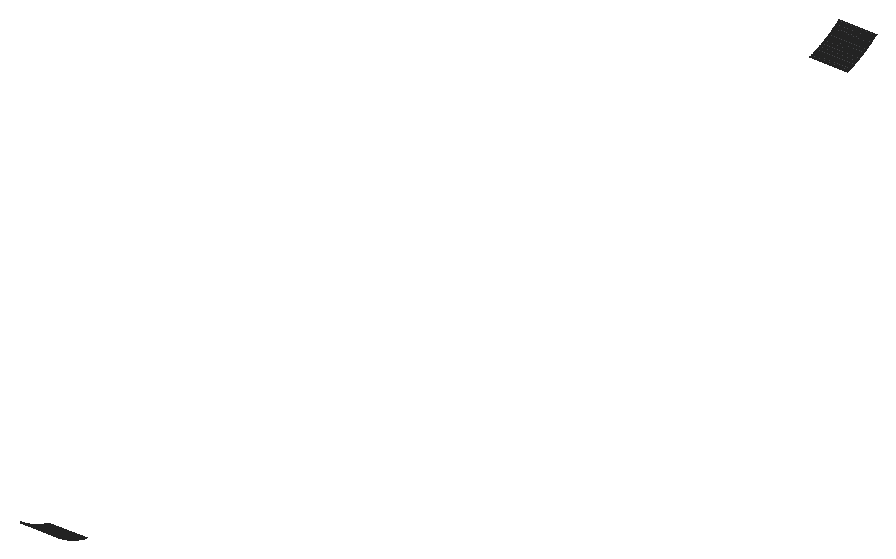
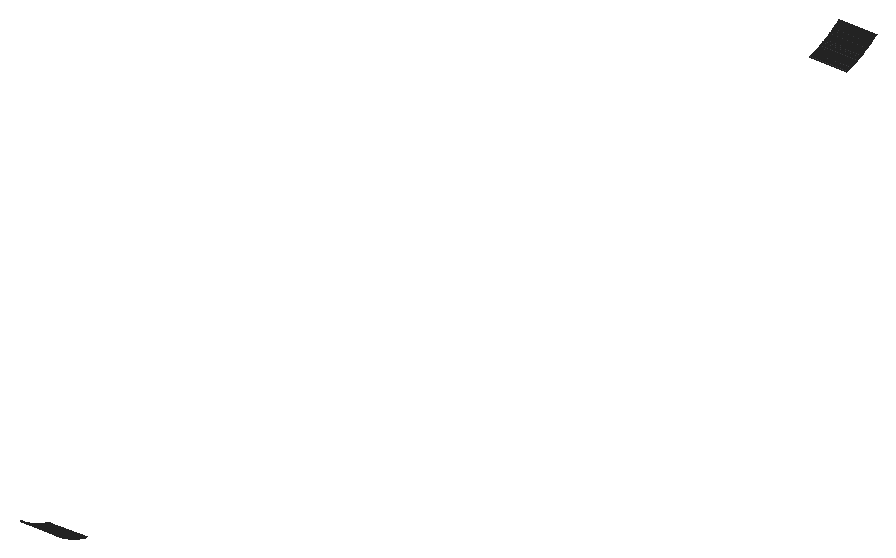
# SketchUp Ruby script. Lengths in inches.
U = 1.inch
M = Sketchup.active_model
def pt(a) = Geom::Point3d.new(a.map { |v| v * U })
def face(e, loops, mat)
  f = e.add_face(loops[0].map { |a| pt(a) })
  loops[1..].each { |l| e.add_face(l.map { |a| pt(a) }).erase! }
  f.material = f.back_material = mat if mat
  f
end
# faces: each face lists its corners as indices into pts; further lists are holes
def faces(e, pts, list, mat = nil) = list.each { |f| face(e, (f[0].is_a?(Array) ? f : [f]).map { |l| l.map { |i| pts[i] } }, mat) }
# xy, xz, yz: faces in a plane at the given z, y or x. An outline is a flat list of corners, or four numbers for a rectangle; further outlines are holes
def ring(l) = l.size == 4 ? [[l[0], l[1]], [l[2], l[1]], [l[2], l[3]], [l[0], l[3]]] : l.each_slice(2).to_a
def flat(e, list, mat, &to3) = list.each { |f| face(e, (f[0].is_a?(Array) ? f : [f]).map { |l| ring(l).map { |u, v| to3.(u, v) } }, mat) }
def xy(e, z, list, mat = nil) = flat(e, list, mat) { |x, y| [x, y, z] }
def xz(e, y, list, mat = nil) = flat(e, list, mat) { |x, z| [x, y, z] }
def yz(e, x, list, mat = nil) = flat(e, list, mat) { |y, z| [x, y, z] }
def lines(e, pts, list) = list.each { |a, b| e.add_line(pt(pts[a]), pt(pts[b])) }
# prism: a flat outline (further loops are holes) pulled along v
def prism(e, loops, v, mat = nil)
  f = face(e, loops, mat); d = Geom::Vector3d.new(v.map { |x| x * U })
  f.pushpull(f.normal.samedirection?(d) ? d.length : -d.length)
end
def box(e, o, s, mat = nil) = prism(e, [[o, [o[0] + s[0], o[1], o[2]], [o[0] + s[0], o[1] + s[1], o[2]], [o[0], o[1] + s[1], o[2]]]], [0, 0, s[2]], mat)
def at(x, y, z, deg = 0) = Geom::Transformation.translation(pt([x, y, z])) * Geom::Transformation.rotation(ORIGIN, Z_AXIS, deg.degrees)
def axes(o, x, y, z) = Geom::Transformation.new([*x, 0, *y, 0, *z, 0, *pt(o).to_a, 1])
def part(name) = M.definitions.add(name)
# library, detail: a bought-in or finely detailed component or shape, given as its bounding box
def library(name, o, s) = part(name).tap { |d| box(d.entities, o, s) }
def detail(e, o, s) = box(e.add_group.entities, o, s)
def put(e, d, t, mat = nil) = e.add_instance(d, t).tap { |i| i.material = mat if mat }
def group(e, t, mat = nil) = e.add_group.tap { |g| g.transformation = t; g.material = mat if mat }.entities
root = M.entities
M.materials.add("1432 AP 8245 TAR ROAD").color = [71, 72, 75]
p = [[573,133.87,145.07],[573,134.14,144.99],[585,134.14,144.99],[585,133.87,145.07],[573,133.33,145.22],[573,133.6,145.14],
  [585,133.6,145.14],[585,133.33,145.22],[573,440.87,145.07],[573,441.14,145.14],[585,441.14,145.14],[585,440.87,145.07],
  [573,441.41,145.22],[585,441.41,145.22],[573,133.06,145.3],[585,133.06,145.3],[573,441.68,145.3],[585,441.68,145.3],
  [573,132.78,145.38],[585,132.78,145.38],[573,441.96,145.38],[585,441.96,145.38],[573,132.51,145.47],[585,132.51,145.47],
  [573,442.23,145.47],[585,442.23,145.47],[573,132.25,145.55],[585,132.25,145.55],[573,442.49,145.55],[585,442.49,145.55],
  [573,131.71,145.73],[573,131.98,145.64],[585,131.98,145.64],[585,131.71,145.73],[573,442.76,145.64],[585,442.76,145.64],
  [573,443.03,145.73],[585,443.03,145.73],[573,131.44,145.83],[585,131.44,145.83],[573,443.3,145.83],[585,443.3,145.83],
  [573,131.18,145.92],[585,131.18,145.92],[573,443.5625,145.92],[585,443.5625,145.92],[573,130.91,146.02],[585,130.91,146.02],
  [573,443.83,146.02],[585,443.83,146.02],[573,130.64,146.12],[585,130.64,146.12],[573,444.1,146.12],[585,444.1,146.12],
  [573,130.38,146.22],[585,130.38,146.22],[573,444.36,146.22],[585,444.36,146.22],[573,130.12,146.32],[585,130.12,146.32],
  [573,444.62,146.32],[585,444.62,146.32],[573,129.85,146.43],[585,129.85,146.43],[573,444.88,146.43],[585,444.88,146.43],
  [573,129.59,146.53],[585,129.59,146.53],[573,445.15,146.53],[585,445.15,146.53],[573,129.33,146.64],[585,129.33,146.64],
  [573,445.41,146.64],[585,445.41,146.64],[573,129.07,146.75],[585,129.07,146.75],[573,445.67,146.75],[585,445.67,146.75],
  [573,128.8125,146.87],[585,128.8125,146.87],[573,445.93,146.87],[585,445.93,146.87],[573,128.56,146.98],[585,128.56,146.98],
  [573,446.18,146.98],[585,446.18,146.98],[573,128.3,147.1],[585,128.3,147.1],[573,446.44,147.1],[585,446.44,147.1],
  [573,128.04,147.22],[585,128.04,147.22],[573,446.7,147.22],[585,446.7,147.22],[573,127.79,147.34],[585,127.79,147.34],
  [573,446.95,147.34],[585,446.95,147.34],[573,127.53,147.46],[585,127.53,147.46],[573,447.21,147.46],[585,447.21,147.46],
  [573,127.28,147.59],[585,127.28,147.59],[573,447.46,147.59],[585,447.46,147.59],[573,127.03,147.72],[585,127.03,147.72],
  [573,447.71,147.72],[585,447.71,147.72],[573,126.77,147.85],[585,126.77,147.85],[573,447.97,147.85],[585,447.97,147.85],
  [573,126.52,147.98],[585,126.52,147.98],[573,448.22,147.98],[585,448.22,147.98],[573,126.28,148.11],[585,126.28,148.11],
  [573,448.46,148.11],[585,448.46,148.11],[573,126.03,148.25],[585,126.03,148.25],[573,448.71,148.25],[585,448.71,148.25],
  [573,125.78,148.38],[585,125.78,148.38],[573,448.96,148.38],[585,448.96,148.38],[573,125.53,148.52],[585,125.53,148.52],
  [573,449.21,148.52],[585,449.21,148.52],[573,125.29,148.66],[585,125.29,148.66],[573,449.45,148.66],[585,449.45,148.66],
  [573,125.04,148.81],[585,125.04,148.81],[573,449.7,148.81],[585,449.7,148.81],[573,124.8,148.95],[585,124.8,148.95],
  [573,449.9375,148.95],[585,449.9375,148.95],[573,124.56,149.1],[585,124.56,149.1],[573,450.18,149.1],[585,450.18,149.1],
  [573,124.32,149.25],[585,124.32,149.25],[573,450.42,149.25],[585,450.42,149.25],[573,124.08,149.4],[585,124.08,149.4],
  [573,450.66,149.4],[585,450.66,149.4],[573,123.84,149.55],[585,123.84,149.55],[573,450.9,149.55],[585,450.9,149.55],
  [573,123.61,149.7],[585,123.61,149.7],[573,451.13,149.7],[585,451.13,149.7],[573,123.37,149.86],[585,123.37,149.86],
  [573,451.37,149.86],[585,451.37,149.86],[573,123.13,150.02],[585,123.13,150.02],[573,451.6,150.02],[585,451.6,150.02],
  [573,122.9,150.18],[585,122.9,150.18],[573,451.84,150.18],[585,451.84,150.18],[573,122.67,150.34],[585,122.67,150.34],
  [573,452.07,150.34],[585,452.07,150.34],[573,122.4375,150.5],[585,122.4375,150.5],[573,452.3,150.5],[585,452.3,150.5],
  [573,452.53,150.67],[585,452.53,150.67]]
faces(root,p,[[0,1,2,3],[4,5,6,7],[5,0,3,6],[8,9,10,11],[9,12,13,10],[14,4,7,15],[12,16,17,13],[18,14,15,19],
  [16,20,21,17],[22,18,19,23],[20,24,25,21],[26,22,23,27],[24,28,29,25],[30,31,32,33],[31,26,27,32],[28,34,35,29],
  [34,36,37,35],[38,30,33,39],[36,40,41,37],[42,38,39,43],[40,44,45,41],[46,42,43,47],[44,48,49,45],[50,46,47,51],
  [48,52,53,49],[54,50,51,55],[52,56,57,53],[58,54,55,59],[56,60,61,57],[62,58,59,63],[60,64,65,61],[66,62,63,67],
  [64,68,69,65],[70,66,67,71],[68,72,73,69],[74,70,71,75],[72,76,77,73],[78,74,75,79],[76,80,81,77],[82,78,79,83],
  [80,84,85,81],[86,82,83,87],[84,88,89,85],[90,86,87,91],[88,92,93,89],[94,90,91,95],[92,96,97,93],[98,94,95,99],
  [96,100,101,97],[102,98,99,103],[100,104,105,101],[106,102,103,107],[104,108,109,105],[110,106,107,111],[108,112,113,109],[114,110,111,115],
  [112,116,117,113],[118,114,115,119],[116,120,121,117],[122,118,119,123],[120,124,125,121],[126,122,123,127],[124,128,129,125],[130,126,127,131],
  [128,132,133,129],[134,130,131,135],[132,136,137,133],[138,134,135,139],[136,140,141,137],[142,138,139,143],[140,144,145,141],[146,142,143,147],
  [144,148,149,145],[150,146,147,151],[148,152,153,149],[154,150,151,155],[152,156,157,153],[158,154,155,159],[156,160,161,157],[162,158,159,163],
  [160,164,165,161],[166,162,163,167],[164,168,169,165],[170,166,167,171],[168,172,173,169],[174,170,171,175],[172,176,177,173],[178,174,175,179],
  [176,180,181,177],[182,178,179,183],[180,184,185,181],[184,186,187,185]],"1432 AP 8245 TAR ROAD")
